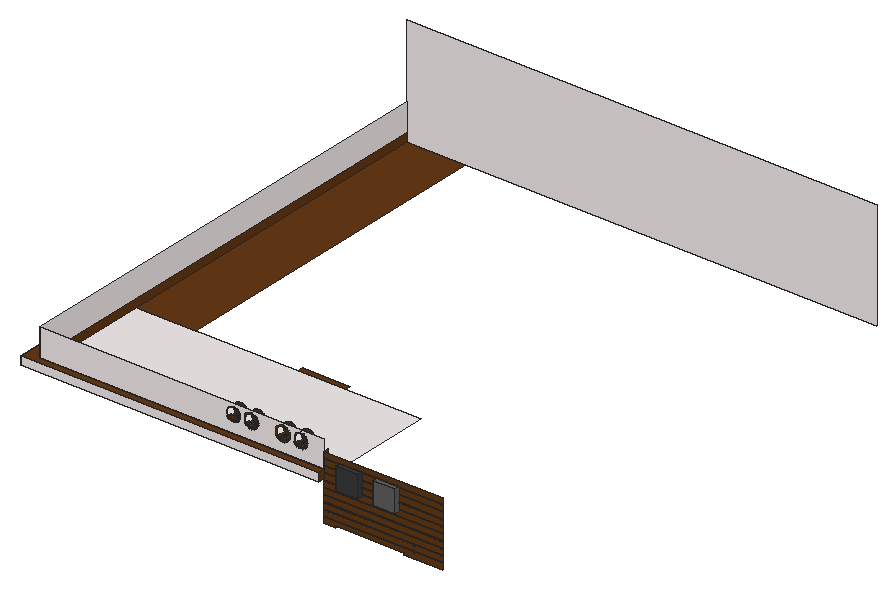
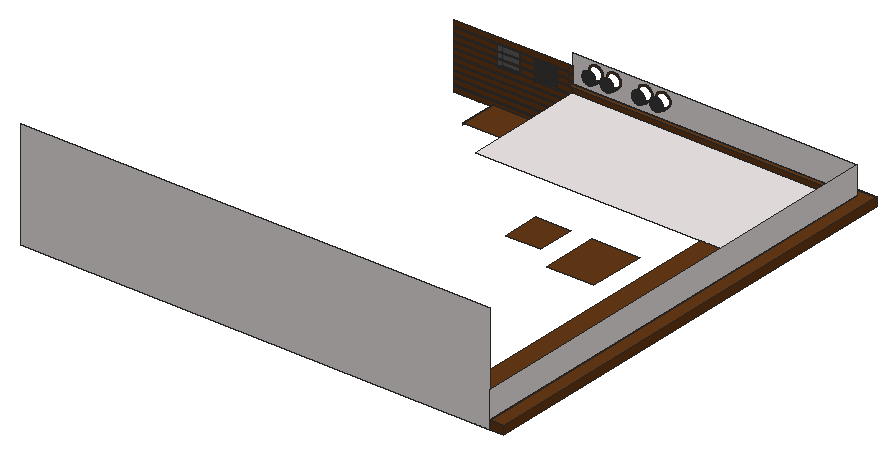
# SketchUp Ruby script. Lengths in inches.
U = 1.inch
M = Sketchup.active_model
def pt(a) = Geom::Point3d.new(a.map { |v| v * U })
def face(e, loops, mat)
  f = e.add_face(loops[0].map { |a| pt(a) })
  loops[1..].each { |l| e.add_face(l.map { |a| pt(a) }).erase! }
  f.material = f.back_material = mat if mat
  f
end
# faces: each face lists its corners as indices into pts; further lists are holes
def faces(e, pts, list, mat = nil) = list.each { |f| face(e, (f[0].is_a?(Array) ? f : [f]).map { |l| l.map { |i| pts[i] } }, mat) }
# xy, xz, yz: faces in a plane at the given z, y or x. An outline is a flat list of corners, or four numbers for a rectangle; further outlines are holes
def ring(l) = l.size == 4 ? [[l[0], l[1]], [l[2], l[1]], [l[2], l[3]], [l[0], l[3]]] : l.each_slice(2).to_a
def flat(e, list, mat, &to3) = list.each { |f| face(e, (f[0].is_a?(Array) ? f : [f]).map { |l| ring(l).map { |u, v| to3.(u, v) } }, mat) }
def xy(e, z, list, mat = nil) = flat(e, list, mat) { |x, y| [x, y, z] }
def xz(e, y, list, mat = nil) = flat(e, list, mat) { |x, z| [x, y, z] }
def yz(e, x, list, mat = nil) = flat(e, list, mat) { |y, z| [x, y, z] }
def lines(e, pts, list) = list.each { |a, b| e.add_line(pt(pts[a]), pt(pts[b])) }
# prism: a flat outline (further loops are holes) pulled along v
def prism(e, loops, v, mat = nil)
  f = face(e, loops, mat); d = Geom::Vector3d.new(v.map { |x| x * U })
  f.pushpull(f.normal.samedirection?(d) ? d.length : -d.length)
end
def box(e, o, s, mat = nil) = prism(e, [[o, [o[0] + s[0], o[1], o[2]], [o[0] + s[0], o[1] + s[1], o[2]], [o[0], o[1] + s[1], o[2]]]], [0, 0, s[2]], mat)
def at(x, y, z, deg = 0) = Geom::Transformation.translation(pt([x, y, z])) * Geom::Transformation.rotation(ORIGIN, Z_AXIS, deg.degrees)
def axes(o, x, y, z) = Geom::Transformation.new([*x, 0, *y, 0, *z, 0, *pt(o).to_a, 1])
def part(name) = M.definitions.add(name)
# library, detail: a bought-in or finely detailed component or shape, given as its bounding box
def library(name, o, s) = part(name).tap { |d| box(d.entities, o, s) }
def detail(e, o, s) = box(e.add_group.entities, o, s)
def put(e, d, t, mat = nil) = e.add_instance(d, t).tap { |i| i.material = mat if mat }
def group(e, t, mat = nil) = e.add_group.tap { |g| g.transformation = t; g.material = mat if mat }.entities
root = M.entities
M.materials.add("Generic").color = [102, 57, 22]
M.materials.add("Generic\#1").color = [96, 96, 96]
M.materials.add("Generic\#2").color = [59, 59, 59]
M.materials.add("Generic\#3").color = [243, 235, 235]
xy(root,372.75,[[366.12,54.375,377.375,54.68],[377.375,54.375,403,54.68]],"Generic")
xy(root,373.92,[[299.81,54.375,366.12,89.74]],"Generic")
xy(root,376.1875,[[129.97,171.5,176.16,226.25],[196.46,171.5,230.03,208.375]],"Generic")
xy(root,378.0625,[[288.56,54.375,377.375,54.68],[377.375,54.375,403,54.68]],"Generic")
xy(root,379.0625,[[288.56,54.375,377.375,54.68],[377.375,54.375,403,54.68]],"Generic")
xy(root,384.375,[[288.56,54.375,377.375,54.68],[377.375,54.375,403,54.68]],"Generic")
xy(root,385.375,[[288.56,54.375,403,54.68]],"Generic")
xy(root,390.6875,[[288.56,54.375,403,54.68]],"Generic")
xy(root,391.6875,[[288.56,54.375,403,54.68]],"Generic")
xy(root,397,[[288.56,54.375,403,54.68]],"Generic")
xy(root,398,[[288.56,54.375,403,54.68]],"Generic")
xy(root,403.3125,[[288.56,54.375,403,54.68]],"Generic")
xy(root,404.3125,[[288.56,54.375,403,54.68]],"Generic")
xy(root,408.375,[[339.38,49.5625,360.7,54.375]],"Generic\#1")
xy(root,408.375,[[303.32,49.5625,324.63,54.375]],"Generic\#2")
xy(root,409.625,[[288.56,54.375,303.32,54.68],[324.63,54.375,339.38,54.68],[360.7,54.375,403,54.68]],"Generic")
xy(root,410.625,[[288.56,54.375,303.32,54.68],[324.63,54.375,339.38,54.68],[360.7,54.375,403,54.68]],"Generic")
xy(root,411.5,[[0,47.4375,0,498.375,13.1875,498.375,13.1875,54.375,288.56,54.375,288.56,47.4375],[13.1875,171.5,70.5625,498.375]],"Generic")
xy(root,411.5,[[13.1875,54.375,288.56,171.5]],"Generic\#3")
xy(root,415.9375,[[288.56,54.375,303.32,54.68],[324.63,54.375,339.38,54.68],[360.7,54.375,403,54.68]],"Generic")
xy(root,416.9375,[[288.56,54.375,303.32,54.68],[324.63,54.375,339.38,54.68],[360.7,54.375,403,54.68]],"Generic")
xy(root,419.5625,[[0,47.4375,288.56,47.4375,288.56,54.375,13.1875,54.375,13.1875,498.375,0,498.375],[13.1875,54.375,288.56,58.5625]],"Generic")
xy(root,422.25,[[288.56,54.375,303.32,54.68],[324.63,54.375,339.38,54.68],[360.7,54.375,403,54.68]],"Generic")
xy(root,423.25,[[288.56,54.375,303.32,54.68],[324.63,54.375,339.38,54.68],[360.7,54.375,403,54.68]],"Generic")
xy(root,428.5625,[[288.56,54.375,303.32,54.68],[324.63,54.375,339.38,54.68],[360.7,54.375,403,54.68]],"Generic")
xy(root,429.13,[[200.27,54.375,201.1,58.5625],[217.64,54.375,218.48,58.5625],[248.2,54.375,249.04,58.5625],[265.58,54.375,266.41,58.5625]],"Generic")
xy(root,429.5625,[[288.56,54.375,303.32,54.68],[324.63,54.375,339.38,54.68],[360.7,54.375,403,54.68]],"Generic")
xy(root,429.6875,[[339.38,49.5625,360.7,54.375]],"Generic\#1")
xy(root,429.6875,[[303.32,49.5625,324.63,54.375]],"Generic\#2")
xy(root,430.04,[[200.32,54.375,201.05,62.9375],[217.69,54.375,218.42,62.9375],[248.26,54.375,248.99,62.9375],[265.63,54.375,266.36,62.9375]],"Generic")
xz(root,47.4375,[[0,411.5,288.56,419.5625]],"Generic\#3")
xz(root,49.5625,[[339.38,408.375,360.7,429.6875]],"Generic\#1")
xz(root,49.5625,[[303.32,408.375,324.63,429.6875]],"Generic\#2")
xz(root,54.375,[[288.56,372.75,299.81,372.75,299.81,373.92,366.12,373.92,366.12,372.75,403,372.75,403,378.0625,288.56,378.0625],[288.56,379.0625,403,384.375],[288.56,385.375,403,390.6875],[288.56,391.6875,403,397],[288.56,398,403,403.3125],
  [288.56,404.3125,403,404.3125,403,409.625,360.7,409.625,360.7,408.375,339.38,408.375,339.38,409.625,324.63,409.625,324.63,408.375,303.32,408.375,303.32,409.625,288.56,409.625],[303.32,409.625,324.63,410.625],[339.38,409.625,360.7,410.625],[288.56,410.625,303.32,415.9375],[324.63,410.625,339.38,415.9375],
  [360.7,410.625,403,415.9375],[13.1875,411.5,288.56,419.5625],[303.32,415.9375,324.63,416.9375],[339.38,415.9375,360.7,416.9375],[288.56,416.9375,303.32,422.25],
  [324.63,416.9375,339.38,422.25],[360.7,416.9375,403,422.25],[303.32,422.25,324.63,423.25],[339.38,422.25,360.7,423.25],[288.56,423.25,303.32,428.5625],
  [324.63,423.25,339.38,428.5625],[360.7,423.25,403,428.5625],[303.32,428.5625,324.63,429.5625],[339.38,428.5625,360.7,429.5625],[[200.27,429.13,201.1,429.13,201.93,429.23,202.75,429.42,203.53,429.71,204.28,430.08,204.98,430.54,205.62,431.08,206.19,431.6875,206.6875,432.36,207.11,433.08,207.4375,433.85,207.68,434.65,207.82,435.47,207.87,436.31,207.82,437.14,207.68,437.97,207.4375,438.77,207.11,439.53,206.6875,440.26,206.19,440.93,205.62,441.54,204.98,442.07,204.28,442.53,203.53,442.91,202.75,443.19,201.93,443.39,201.1,443.48,200.27,443.48,199.4375,443.39,198.62,443.19,197.84,442.91,197.09,442.53,196.39,442.07,195.75,441.54,195.18,440.93,194.68,440.26,194.26,439.53,193.93,438.77,193.69,437.97,193.55,437.14,193.5,436.31,193.55,435.47,193.69,434.65,193.93,433.85,194.26,433.08,194.68,432.36,195.18,431.6875,195.75,431.08,196.39,430.54,197.09,430.08,197.84,429.71,198.62,429.42,199.4375,429.23],[200.32,430.04,199.59,430.12,198.88,430.29,198.2,430.54,197.54,430.87,196.93,431.27,196.37,431.74,195.87,432.27,195.44,432.86,195.07,433.49,194.78,434.16,194.57,434.86,194.44,435.58,194.4,436.31,194.44,437.04,194.57,437.76,194.78,438.46,195.07,439.13,195.44,439.76,195.87,440.35,196.37,440.88,196.93,441.35,197.54,441.75,198.2,442.08,198.88,442.33,199.59,442.5,200.32,442.58,201.05,442.58,201.78,442.5,202.49,442.33,203.17,442.08,203.83,441.75,204.4375,441.35,205,440.88,205.5,440.35,205.93,439.76,206.3,439.13,206.59,438.46,206.8,437.76,206.92,437.04,206.97,436.31,206.92,435.58,206.8,434.86,206.59,434.16,206.3,433.49,205.93,432.86,205.5,432.27,205,431.74,204.4375,431.27,203.83,430.87,203.17,430.54,202.49,430.29,201.78,430.12,201.05,430.04]],
  [[217.64,429.13,218.48,429.13,219.31,429.23,220.12,429.42,220.91,429.71,221.65,430.08,222.35,430.54,222.99,431.08,223.57,431.6875,224.0625,432.36,224.48,433.08,224.8125,433.85,225.05,434.65,225.2,435.47,225.25,436.31,225.2,437.14,225.05,437.97,224.8125,438.77,224.48,439.53,224.0625,440.26,223.57,440.93,222.99,441.54,222.35,442.07,221.65,442.53,220.91,442.91,220.12,443.19,219.31,443.39,218.48,443.48,217.64,443.48,216.8125,443.39,216,443.19,215.21,442.91,214.47,442.53,213.77,442.07,213.125,441.54,212.55,440.93,212.05,440.26,211.64,439.53,211.31,438.77,211.07,437.97,210.92,437.14,210.87,436.31,210.92,435.47,211.07,434.65,211.31,433.85,211.64,433.08,212.05,432.36,212.55,431.6875,213.125,431.08,213.77,430.54,214.47,430.08,215.21,429.71,216,429.42,216.8125,429.23],[217.69,430.04,216.97,430.12,216.26,430.29,215.57,430.54,214.92,430.87,214.31,431.27,213.75,431.74,213.25,432.27,212.81,432.86,212.44,433.49,212.16,434.16,211.95,434.86,211.82,435.58,211.78,436.31,211.82,437.04,211.95,437.76,212.16,438.46,212.44,439.13,212.81,439.76,213.25,440.35,213.75,440.88,214.31,441.35,214.92,441.75,215.57,442.08,216.26,442.33,216.97,442.5,217.69,442.58,218.42,442.58,219.15,442.5,219.86,442.33,220.55,442.08,221.2,441.75,221.8125,441.35,222.37,440.88,222.87,440.35,223.31,439.76,223.67,439.13,223.96,438.46,224.17,437.76,224.3,437.04,224.34,436.31,224.3,435.58,224.17,434.86,223.96,434.16,223.67,433.49,223.31,432.86,222.87,432.27,222.37,431.74,221.8125,431.27,221.2,430.87,220.55,430.54,219.86,430.29,219.15,430.12,218.42,430.04]],[[248.2,429.13,249.04,429.13,249.87,429.23,250.68,429.42,251.47,429.71,252.22,430.08,252.91,430.54,253.55,431.08,254.13,431.6875,254.625,432.36,255.04,433.08,255.375,433.85,255.62,434.65,255.76,435.47,255.81,436.31,255.76,437.14,255.62,437.97,255.375,438.77,255.04,439.53,254.625,440.26,254.13,440.93,253.55,441.54,252.91,442.07,252.22,442.53,251.47,442.91,250.68,443.19,249.87,443.39,249.04,443.48,248.2,443.48,247.375,443.39,246.56,443.19,245.77,442.91,245.03,442.53,244.33,442.07,243.6875,441.54,243.12,440.93,242.62,440.26,242.2,439.53,241.87,438.77,241.63,437.97,241.48,437.14,241.43,436.31,241.48,435.47,241.63,434.65,241.87,433.85,242.2,433.08,242.62,432.36,243.12,431.6875,243.6875,431.08,244.33,430.54,245.03,430.08,245.77,429.71,246.56,429.42,247.375,429.23],[248.26,430.04,247.53,430.12,246.82,430.29,246.13,430.54,245.48,430.87,244.87,431.27,244.31,431.74,243.81,432.27,243.37,432.86,243.01,433.49,242.72,434.16,242.51,434.86,242.38,435.58,242.34,436.31,242.38,437.04,242.51,437.76,242.72,438.46,243.01,439.13,243.37,439.76,243.81,440.35,244.31,440.88,244.87,441.35,245.48,441.75,246.13,442.08,246.82,442.33,247.53,442.5,248.26,442.58,248.99,442.58,249.71,442.5,250.42,442.33,251.11,442.08,251.76,441.75,252.375,441.35,252.93,440.88,253.43,440.35,253.87,439.76,254.24,439.13,254.53,438.46,254.73,437.76,254.86,437.04,254.9,436.31,254.86,435.58,254.73,434.86,254.53,434.16,254.24,433.49,253.87,432.86,253.43,432.27,252.93,431.74,252.375,431.27,251.76,430.87,251.11,430.54,250.42,430.29,249.71,430.12,248.99,430.04]],[[265.58,429.13,266.41,429.13,267.24,429.23,268.06,429.42,268.84,429.71,269.59,430.08,270.29,430.54,270.93,431.08,271.5,431.6875,272,432.36,272.42,433.08,272.75,433.85,272.99,434.65,273.14,435.47,273.18,436.31,273.14,437.14,272.99,437.97,272.75,438.77,272.42,439.53,272,440.26,271.5,440.93,270.93,441.54,270.29,442.07,269.59,442.53,268.84,442.91,268.06,443.19,267.24,443.39,266.41,443.48,265.58,443.48,264.75,443.39,263.94,443.19,263.15,442.91,262.4,442.53,261.7,442.07,261.0625,441.54,260.49,440.93,259.99,440.26,259.57,439.53,259.24,438.77,259,437.97,258.86,437.14,258.81,436.31,258.86,435.47,259,434.65,259.24,433.85,259.57,433.08,259.99,432.36,260.49,431.6875,261.0625,431.08,261.7,430.54,262.4,430.08,263.15,429.71,263.94,429.42,264.75,429.23],[265.63,430.04,264.91,430.12,264.19,430.29,263.51,430.54,262.86,430.87,262.25,431.27,261.69,431.74,261.18,432.27,260.75,432.86,260.38,433.49,260.09,434.16,259.88,434.86,259.76,435.58,259.71,436.31,259.76,437.04,259.88,437.76,260.09,438.46,260.38,439.13,260.75,439.76,261.18,440.35,261.69,440.88,262.25,441.35,262.86,441.75,263.51,442.08,264.19,442.33,264.91,442.5,265.63,442.58,266.36,442.58,267.09,442.5,267.8,442.33,268.48,442.08,269.14,441.75,269.75,441.35,270.31,440.88,270.81,440.35,271.25,439.76,271.61,439.13,271.9,438.46,272.11,437.76,272.24,437.04,272.28,436.31,272.24,435.58,272.11,434.86,271.9,434.16,271.61,433.49,271.25,432.86,270.81,432.27,270.31,431.74,269.75,431.27,269.14,430.87,268.48,430.54,267.8,430.29,267.09,430.12,266.36,430.04]],[288.56,429.5625,303.32,429.5625,303.32,429.6875,324.63,429.6875,324.63,429.5625,339.38,429.5625,339.38,429.6875,360.7,429.6875,360.7,429.5625,403,429.5625,403,434.875,288.56,434.875]],"Generic")
xz(root,54.375,[[[13.1875,419.5625,288.56,446.16],[265.58,429.13,264.75,429.23,263.94,429.42,263.15,429.71,262.4,430.08,261.7,430.54,261.0625,431.08,260.49,431.6875,259.99,432.36,259.57,433.08,259.24,433.85,259,434.65,258.86,435.47,258.81,436.31,258.86,437.14,259,437.97,259.24,438.77,259.57,439.53,259.99,440.26,260.49,440.93,261.0625,441.54,261.7,442.07,262.4,442.53,263.15,442.91,263.94,443.19,264.75,443.39,265.58,443.48,266.41,443.48,267.24,443.39,268.06,443.19,268.84,442.91,269.59,442.53,270.29,442.07,270.93,441.54,271.5,440.93,272,440.26,272.42,439.53,272.75,438.77,272.99,437.97,273.14,437.14,273.18,436.31,273.14,435.47,272.99,434.65,272.75,433.85,272.42,433.08,272,432.36,271.5,431.6875,270.93,431.08,270.29,430.54,269.59,430.08,268.84,429.71,268.06,429.42,267.24,429.23,266.41,429.13],[217.64,429.13,216.8125,429.23,216,429.42,215.21,429.71,214.47,430.08,213.77,430.54,213.125,431.08,212.55,431.6875,212.05,432.36,211.64,433.08,211.31,433.85,211.07,434.65,210.92,435.47,210.87,436.31,210.92,437.14,211.07,437.97,211.31,438.77,211.64,439.53,212.05,440.26,212.55,440.93,213.125,441.54,213.77,442.07,214.47,442.53,215.21,442.91,216,443.19,216.8125,443.39,217.64,443.48,218.48,443.48,219.31,443.39,220.12,443.19,220.91,442.91,221.65,442.53,222.35,442.07,222.99,441.54,223.57,440.93,224.0625,440.26,224.48,439.53,224.8125,438.77,225.05,437.97,225.2,437.14,225.25,436.31,225.2,435.47,225.05,434.65,224.8125,433.85,224.48,433.08,224.0625,432.36,223.57,431.6875,222.99,431.08,222.35,430.54,221.65,430.08,220.91,429.71,220.12,429.42,219.31,429.23,218.48,429.13],[200.27,429.13,199.4375,429.23,198.62,429.42,197.84,429.71,197.09,430.08,196.39,430.54,195.75,431.08,195.18,431.6875,194.68,432.36,194.26,433.08,193.93,433.85,193.69,434.65,193.55,435.47,193.5,436.31,193.55,437.14,193.69,437.97,193.93,438.77,194.26,439.53,194.68,440.26,195.18,440.93,195.75,441.54,196.39,442.07,197.09,442.53,197.84,442.91,198.62,443.19,199.4375,443.39,200.27,443.48,201.1,443.48,201.93,443.39,202.75,443.19,203.53,442.91,204.28,442.53,204.98,442.07,205.62,441.54,206.19,440.93,206.6875,440.26,207.11,439.53,207.4375,438.77,207.68,437.97,207.82,437.14,207.87,436.31,207.82,435.47,207.68,434.65,207.4375,433.85,207.11,433.08,206.6875,432.36,206.19,431.6875,205.62,431.08,204.98,430.54,204.28,430.08,203.53,429.71,202.75,429.42,201.93,429.23,201.1,429.13],[248.2,429.13,247.375,429.23,246.56,429.42,245.77,429.71,245.03,430.08,244.33,430.54,243.6875,431.08,243.12,431.6875,242.62,432.36,242.2,433.08,241.87,433.85,241.63,434.65,241.48,435.47,241.43,436.31,241.48,437.14,241.63,437.97,241.87,438.77,242.2,439.53,242.62,440.26,243.12,440.93,243.6875,441.54,244.33,442.07,245.03,442.53,245.77,442.91,246.56,443.19,247.375,443.39,248.2,443.48,249.04,443.48,249.87,443.39,250.68,443.19,251.47,442.91,252.22,442.53,252.91,442.07,253.55,441.54,254.13,440.93,254.625,440.26,255.04,439.53,255.375,438.77,255.62,437.97,255.76,437.14,255.81,436.31,255.76,435.47,255.62,434.65,255.375,433.85,255.04,433.08,254.625,432.36,254.13,431.6875,253.55,431.08,252.91,430.54,252.22,430.08,251.47,429.71,250.68,429.42,249.87,429.23,249.04,429.13]]],"Generic\#3")
xz(root,54.68,[[288.56,378.0625,403,379.0625],[288.56,384.375,403,385.375],[288.56,390.6875,403,391.6875],[288.56,397,403,398],[288.56,403.3125,403,404.3125],
  [288.56,409.625,303.32,410.625],[324.63,409.625,339.38,410.625],[360.7,409.625,403,410.625],[288.56,415.9375,303.32,416.9375],[324.63,415.9375,339.38,416.9375],
  [360.7,415.9375,403,416.9375],[288.56,422.25,303.32,423.25],[324.63,422.25,339.38,423.25],[360.7,422.25,403,423.25],[288.56,428.5625,303.32,429.5625],
  [324.63,428.5625,339.38,429.5625],[360.7,428.5625,403,429.5625]],"Generic")
xz(root,62.9375,[[200.32,430.04,201.05,430.04,201.78,430.12,202.49,430.29,203.17,430.54,203.83,430.87,204.4375,431.27,205,431.74,205.5,432.27,205.93,432.86,206.3,433.49,206.59,434.16,206.8,434.86,206.92,435.58,206.97,436.31,206.92,437.04,206.8,437.76,206.59,438.46,206.3,439.13,205.93,439.76,205.5,440.35,205,440.88,204.4375,441.35,203.83,441.75,203.17,442.08,202.49,442.33,201.78,442.5,201.05,442.58,200.32,442.58,199.59,442.5,198.88,442.33,198.2,442.08,197.54,441.75,196.93,441.35,196.37,440.88,195.87,440.35,195.44,439.76,195.07,439.13,194.78,438.46,194.57,437.76,194.44,437.04,194.4,436.31,194.44,435.58,194.57,434.86,194.78,434.16,195.07,433.49,195.44,432.86,195.87,432.27,196.37,431.74,196.93,431.27,197.54,430.87,198.2,430.54,198.88,430.29,199.59,430.12],[217.69,430.04,218.42,430.04,219.15,430.12,219.86,430.29,220.55,430.54,221.2,430.87,221.8125,431.27,222.37,431.74,222.87,432.27,223.31,432.86,223.67,433.49,223.96,434.16,224.17,434.86,224.3,435.58,224.34,436.31,224.3,437.04,224.17,437.76,223.96,438.46,223.67,439.13,223.31,439.76,222.87,440.35,222.37,440.88,221.8125,441.35,221.2,441.75,220.55,442.08,219.86,442.33,219.15,442.5,218.42,442.58,217.69,442.58,216.97,442.5,216.26,442.33,215.57,442.08,214.92,441.75,214.31,441.35,213.75,440.88,213.25,440.35,212.81,439.76,212.44,439.13,212.16,438.46,211.95,437.76,211.82,437.04,211.78,436.31,211.82,435.58,211.95,434.86,212.16,434.16,212.44,433.49,212.81,432.86,213.25,432.27,213.75,431.74,214.31,431.27,214.92,430.87,215.57,430.54,216.26,430.29,216.97,430.12],[248.26,430.04,248.99,430.04,249.71,430.12,250.42,430.29,251.11,430.54,251.76,430.87,252.375,431.27,252.93,431.74,253.43,432.27,253.87,432.86,254.24,433.49,254.53,434.16,254.73,434.86,254.86,435.58,254.9,436.31,254.86,437.04,254.73,437.76,254.53,438.46,254.24,439.13,253.87,439.76,253.43,440.35,252.93,440.88,252.375,441.35,251.76,441.75,251.11,442.08,250.42,442.33,249.71,442.5,248.99,442.58,248.26,442.58,247.53,442.5,246.82,442.33,246.13,442.08,245.48,441.75,244.87,441.35,244.31,440.88,243.81,440.35,243.37,439.76,243.01,439.13,242.72,438.46,242.51,437.76,242.38,437.04,242.34,436.31,242.38,435.58,242.51,434.86,242.72,434.16,243.01,433.49,243.37,432.86,243.81,432.27,244.31,431.74,244.87,431.27,245.48,430.87,246.13,430.54,246.82,430.29,247.53,430.12],[265.63,430.04,266.36,430.04,267.09,430.12,267.8,430.29,268.48,430.54,269.14,430.87,269.75,431.27,270.31,431.74,270.81,432.27,271.25,432.86,271.61,433.49,271.9,434.16,272.11,434.86,272.24,435.58,272.28,436.31,272.24,437.04,272.11,437.76,271.9,438.46,271.61,439.13,271.25,439.76,270.81,440.35,270.31,440.88,269.75,441.35,269.14,441.75,268.48,442.08,267.8,442.33,267.09,442.5,266.36,442.58,265.63,442.58,264.91,442.5,264.19,442.33,263.51,442.08,262.86,441.75,262.25,441.35,261.69,440.88,261.18,440.35,260.75,439.76,260.38,439.13,260.09,438.46,259.88,437.76,259.76,437.04,259.71,436.31,259.76,435.58,259.88,434.86,260.09,434.16,260.38,433.49,260.75,432.86,261.18,432.27,261.69,431.74,262.25,431.27,262.86,430.87,263.51,430.54,264.19,430.29,264.91,430.12]],"Generic\#2")
xz(root,498.375,[[0,411.5,13.1875,419.5625]],"Generic")
xz(root,498.375,[[13.1875,411.5,467.875,517.125]],"Generic\#3")
yz(root,0,[[47.4375,411.5,498.375,419.5625]],"Generic")
yz(root,13.1875,[[54.375,411.5,498.375,419.5625]],"Generic")
yz(root,13.1875,[[54.375,419.5625,498.375,446.16]],"Generic\#3")
yz(root,288.56,[[47.4375,411.5,54.375,419.5625],[54.375,415.9375,54.68,416.9375],[54.375,419.5625,58.5625,422.25],[54.375,422.25,54.68,423.25],[54.68,422.25,58.5625,423.25],
  [54.375,423.25,58.5625,428.5625],[54.375,428.5625,54.68,429.5625],[54.68,428.5625,58.5625,429.5625],[54.375,429.5625,58.5625,434.875]],"Generic")
yz(root,299.81,[[54.375,372.75,89.74,373.92]],"Generic")
yz(root,303.32,[[54.375,409.625,54.68,410.625],[54.375,415.9375,54.68,416.9375],[54.375,422.25,54.68,423.25],[54.375,428.5625,54.68,429.5625]],"Generic")
yz(root,303.32,[[49.5625,408.375,54.375,429.6875]],"Generic\#2")
yz(root,324.63,[[54.375,409.625,54.68,410.625],[54.375,415.9375,54.68,416.9375],[54.375,422.25,54.68,423.25],[54.375,428.5625,54.68,429.5625]],"Generic")
yz(root,324.63,[[49.5625,408.375,54.375,429.6875]],"Generic\#2")
yz(root,339.38,[[54.375,409.625,54.68,410.625],[54.375,415.9375,54.68,416.9375],[54.375,422.25,54.68,423.25],[54.375,428.5625,54.68,429.5625]],"Generic")
yz(root,339.38,[[49.5625,408.375,54.375,429.6875]],"Generic\#1")
yz(root,360.7,[[54.375,409.625,54.68,410.625],[54.375,415.9375,54.68,416.9375],[54.375,422.25,54.68,423.25],[54.375,428.5625,54.68,429.5625]],"Generic")
yz(root,360.7,[[49.5625,408.375,54.375,429.6875]],"Generic\#1")
yz(root,366.12,[[54.375,372.75,89.74,373.92]],"Generic")
yz(root,403,[[54.375,378.0625,54.68,379.0625],[54.375,384.375,54.68,385.375],[54.375,390.6875,54.68,391.6875],[54.375,397,54.68,398],[54.375,403.3125,54.68,404.3125],
  [54.375,409.625,54.68,410.625],[54.375,415.9375,54.68,416.9375],[54.375,422.25,54.68,423.25],[54.375,428.5625,54.68,429.5625]],"Generic")
p = [[199.4375,54.375,429.23],[200.27,54.375,429.13],[200.27,58.5625,429.13],[199.4375,58.5625,429.23],[201.1,54.375,429.13],[201.93,54.375,429.23],
  [201.93,58.5625,429.23],[201.1,58.5625,429.13],[216.8125,54.375,429.23],[217.64,54.375,429.13],[217.64,58.5625,429.13],[216.8125,58.5625,429.23],
  [218.48,54.375,429.13],[219.31,54.375,429.23],[219.31,58.5625,429.23],[218.48,58.5625,429.13],[247.375,54.375,429.23],[248.2,54.375,429.13],
  [248.2,58.5625,429.13],[247.375,58.5625,429.23],[249.04,54.375,429.13],[249.87,54.375,429.23],[249.87,58.5625,429.23],[249.04,58.5625,429.13],
  [264.75,54.375,429.23],[265.58,54.375,429.13],[265.58,58.5625,429.13],[264.75,58.5625,429.23],[266.41,54.375,429.13],[267.24,54.375,429.23],
  [267.24,58.5625,429.23],[266.41,58.5625,429.13],[198.62,54.375,429.42],[198.62,58.5625,429.42],[202.75,54.375,429.42],[202.75,58.5625,429.42],
  [216,54.375,429.42],[216,58.5625,429.42],[220.12,54.375,429.42],[220.12,58.5625,429.42],[246.56,54.375,429.42],[246.56,58.5625,429.42],
  [250.68,54.375,429.42],[250.68,58.5625,429.42],[263.94,54.375,429.42],[263.94,58.5625,429.42],[268.06,54.375,429.42],[268.06,58.5625,429.42],
  [197.84,54.375,429.71],[197.84,58.5625,429.71],[203.53,54.375,429.71],[203.53,58.5625,429.71],[215.21,54.375,429.71],[215.21,58.5625,429.71],
  [220.91,54.375,429.71],[220.91,58.5625,429.71],[245.77,54.375,429.71],[245.77,58.5625,429.71],[251.47,54.375,429.71],[251.47,58.5625,429.71],
  [263.15,54.375,429.71],[263.15,58.5625,429.71],[268.84,54.375,429.71],[268.84,58.5625,429.71],[197.09,54.375,430.08],[197.09,58.5625,430.08],
  [204.28,54.375,430.08],[204.28,58.5625,430.08],[214.47,54.375,430.08],[214.47,58.5625,430.08],[221.65,54.375,430.08],[221.65,58.5625,430.08],
  [245.03,54.375,430.08],[245.03,58.5625,430.08],[252.22,54.375,430.08],[252.22,58.5625,430.08],[262.4,54.375,430.08],[262.4,58.5625,430.08],
  [269.59,54.375,430.08],[269.59,58.5625,430.08],[199.59,54.375,430.12],[200.32,54.375,430.04],[200.32,62.9375,430.04],[199.59,62.9375,430.12],
  [201.05,54.375,430.04],[201.78,54.375,430.12],[201.78,62.9375,430.12],[201.05,62.9375,430.04],[216.97,54.375,430.12],[217.69,54.375,430.04],
  [217.69,62.9375,430.04],[216.97,62.9375,430.12],[218.42,54.375,430.04],[219.15,54.375,430.12],[219.15,62.9375,430.12],[218.42,62.9375,430.04],
  [247.53,54.375,430.12],[248.26,54.375,430.04],[248.26,62.9375,430.04],[247.53,62.9375,430.12],[248.99,54.375,430.04],[249.71,54.375,430.12],
  [249.71,62.9375,430.12],[248.99,62.9375,430.04],[264.91,54.375,430.12],[265.63,54.375,430.04],[265.63,62.9375,430.04],[264.91,62.9375,430.12],
  [266.36,54.375,430.04],[267.09,54.375,430.12],[267.09,62.9375,430.12],[266.36,62.9375,430.04],[196.39,54.375,430.54],[196.39,58.5625,430.54],
  [198.88,54.375,430.29],[198.88,62.9375,430.29],[202.49,54.375,430.29],[202.49,62.9375,430.29],[204.98,54.375,430.54],[204.98,58.5625,430.54],
  [213.77,54.375,430.54],[213.77,58.5625,430.54],[216.26,54.375,430.29],[216.26,62.9375,430.29],[219.86,54.375,430.29],[219.86,62.9375,430.29],
  [222.35,54.375,430.54],[222.35,58.5625,430.54],[244.33,54.375,430.54],[244.33,58.5625,430.54],[246.82,54.375,430.29],[246.82,62.9375,430.29],
  [250.42,54.375,430.29],[250.42,62.9375,430.29],[252.91,54.375,430.54],[252.91,58.5625,430.54],[261.7,54.375,430.54],[261.7,58.5625,430.54],
  [264.19,54.375,430.29],[264.19,62.9375,430.29],[267.8,54.375,430.29],[267.8,62.9375,430.29],[270.29,54.375,430.54],[270.29,58.5625,430.54],
  [198.2,54.375,430.54],[198.2,62.9375,430.54],[203.17,54.375,430.54],[203.17,62.9375,430.54],[215.57,54.375,430.54],[215.57,62.9375,430.54],
  [220.55,54.375,430.54],[220.55,62.9375,430.54],[246.13,54.375,430.54],[246.13,62.9375,430.54],[251.11,54.375,430.54],[251.11,62.9375,430.54],
  [263.51,54.375,430.54],[263.51,62.9375,430.54],[268.48,54.375,430.54],[268.48,62.9375,430.54],[195.75,54.375,431.08],[195.75,58.5625,431.08],
  [197.54,54.375,430.87],[197.54,62.9375,430.87],[203.83,54.375,430.87],[203.83,62.9375,430.87],[205.62,54.375,431.08],[205.62,58.5625,431.08],
  [213.125,54.375,431.08],[213.125,58.5625,431.08],[214.92,54.375,430.87],[214.92,62.9375,430.87],[221.2,54.375,430.87],[221.2,62.9375,430.87],
  [222.99,54.375,431.08],[222.99,58.5625,431.08],[243.6875,54.375,431.08],[243.6875,58.5625,431.08],[245.48,54.375,430.87],[245.48,62.9375,430.87],
  [251.76,54.375,430.87],[251.76,62.9375,430.87],[253.55,54.375,431.08],[253.55,58.5625,431.08],[261.0625,54.375,431.08],[261.0625,58.5625,431.08],
  [262.86,54.375,430.87],[262.86,62.9375,430.87],[269.14,54.375,430.87],[269.14,62.9375,430.87],[270.93,54.375,431.08],[270.93,58.5625,431.08],
  [196.93,54.375,431.27],[196.93,62.9375,431.27],[204.4375,54.375,431.27],[204.4375,62.9375,431.27],[214.31,54.375,431.27],[214.31,62.9375,431.27],
  [221.8125,54.375,431.27],[221.8125,62.9375,431.27],[244.87,54.375,431.27],[244.87,62.9375,431.27],[252.375,54.375,431.27],[252.375,62.9375,431.27],
  [262.25,54.375,431.27],[262.25,62.9375,431.27],[269.75,54.375,431.27],[269.75,62.9375,431.27],[195.18,54.375,431.6875],[195.18,58.5625,431.6875],
  [206.19,54.375,431.6875],[206.19,58.5625,431.6875],[212.55,54.375,431.6875],[212.55,58.5625,431.6875],[223.57,54.375,431.6875],[223.57,58.5625,431.6875],
  [243.12,54.375,431.6875],[243.12,58.5625,431.6875],[254.13,54.375,431.6875],[254.13,58.5625,431.6875],[260.49,54.375,431.6875],[260.49,58.5625,431.6875],
  [271.5,54.375,431.6875],[271.5,58.5625,431.6875],[196.37,54.375,431.74],[196.37,62.9375,431.74],[205,54.375,431.74],[205,62.9375,431.74],
  [213.75,54.375,431.74],[213.75,62.9375,431.74],[222.37,54.375,431.74],[222.37,62.9375,431.74],[244.31,54.375,431.74],[244.31,62.9375,431.74],
  [252.93,54.375,431.74],[252.93,62.9375,431.74],[261.69,54.375,431.74],[261.69,62.9375,431.74],[270.31,54.375,431.74],[270.31,62.9375,431.74],
  [194.68,54.375,432.36],[194.68,58.5625,432.36],[195.87,54.375,432.27],[195.87,62.9375,432.27],[205.5,54.375,432.27],[205.5,62.9375,432.27],
  [206.6875,54.375,432.36],[206.6875,58.5625,432.36],[212.05,54.375,432.36],[212.05,58.5625,432.36],[213.25,54.375,432.27],[213.25,62.9375,432.27],
  [222.87,54.375,432.27],[222.87,62.9375,432.27],[224.0625,54.375,432.36],[224.0625,58.5625,432.36],[242.62,54.375,432.36],[242.62,58.5625,432.36],
  [243.81,54.375,432.27],[243.81,62.9375,432.27],[253.43,54.375,432.27],[253.43,62.9375,432.27],[254.625,54.375,432.36],[254.625,58.5625,432.36],
  [259.99,54.375,432.36],[259.99,58.5625,432.36],[261.18,54.375,432.27],[261.18,62.9375,432.27],[270.81,54.375,432.27],[270.81,62.9375,432.27],
  [272,54.375,432.36],[272,58.5625,432.36]]
faces(root,p,[[0,1,2,3],[4,5,6,7],[8,9,10,11],[12,13,14,15],[16,17,18,19],[20,21,22,23],[24,25,26,27],[28,29,30,31],
  [32,0,3,33],[5,34,35,6],[36,8,11,37],[13,38,39,14],[40,16,19,41],[21,42,43,22],[44,24,27,45],[29,46,47,30],
  [48,32,33,49],[34,50,51,35],[52,36,37,53],[38,54,55,39],[56,40,41,57],[42,58,59,43],[60,44,45,61],[46,62,63,47],
  [64,48,49,65],[50,66,67,51],[68,52,53,69],[54,70,71,55],[72,56,57,73],[58,74,75,59],[76,60,61,77],[62,78,79,63],
  [80,81,82,83],[84,85,86,87],[88,89,90,91],[92,93,94,95],[96,97,98,99],[100,101,102,103],[104,105,106,107],[108,109,110,111],
  [112,64,65,113],[114,80,83,115],[85,116,117,86],[66,118,119,67],[120,68,69,121],[122,88,91,123],[93,124,125,94],[70,126,127,71],
  [128,72,73,129],[130,96,99,131],[101,132,133,102],[74,134,135,75],[136,76,77,137],[138,104,107,139],[109,140,141,110],[78,142,143,79],
  [144,114,115,145],[116,146,147,117],[148,122,123,149],[124,150,151,125],[152,130,131,153],[132,154,155,133],[156,138,139,157],[140,158,159,141],
  [160,112,113,161],[162,144,145,163],[146,164,165,147],[118,166,167,119],[168,120,121,169],[170,148,149,171],[150,172,173,151],[126,174,175,127],
  [176,128,129,177],[178,152,153,179],[154,180,181,155],[134,182,183,135],[184,136,137,185],[186,156,157,187],[158,188,189,159],[142,190,191,143],
  [192,162,163,193],[164,194,195,165],[196,170,171,197],[172,198,199,173],[200,178,179,201],[180,202,203,181],[204,186,187,205],[188,206,207,189],
  [208,160,161,209],[166,210,211,167],[212,168,169,213],[174,214,215,175],[216,176,177,217],[182,218,219,183],[220,184,185,221],[190,222,223,191],
  [224,192,193,225],[194,226,227,195],[228,196,197,229],[198,230,231,199],[232,200,201,233],[202,234,235,203],[236,204,205,237],[206,238,239,207],
  [240,208,209,241],[242,224,225,243],[226,244,245,227],[210,246,247,211],[248,212,213,249],[250,228,229,251],[230,252,253,231],[214,254,255,215],
  [256,216,217,257],[258,232,233,259],[234,260,261,235],[218,262,263,219],[264,220,221,265],[266,236,237,267],[238,268,269,239],[222,270,271,223]],"Generic")
